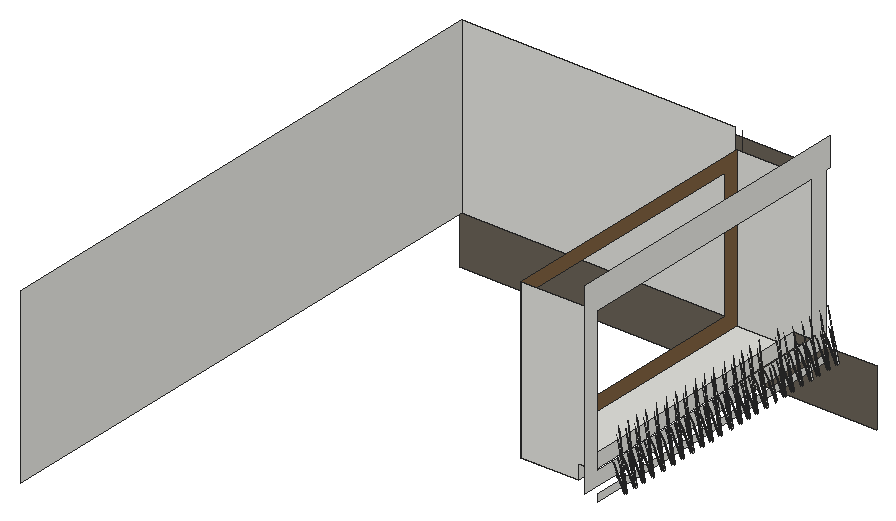
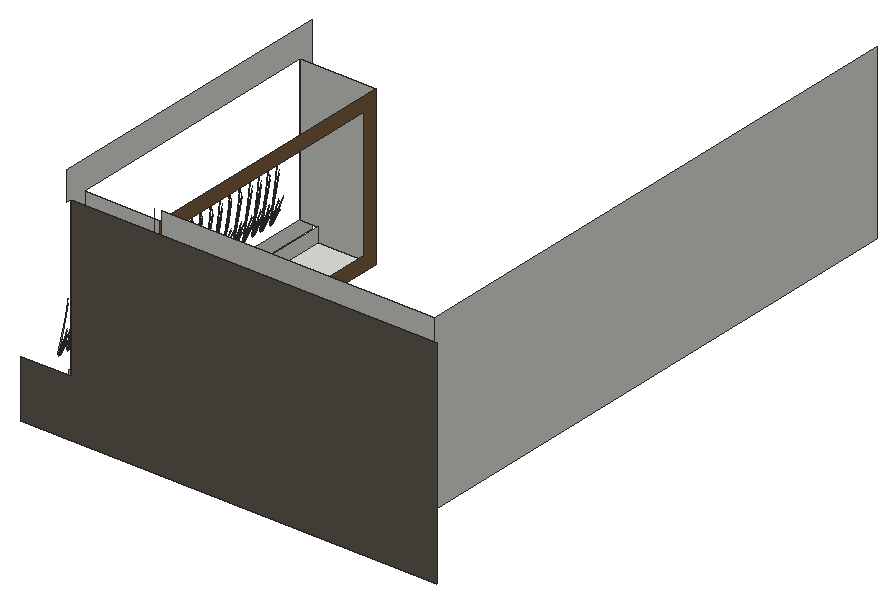
# SketchUp Ruby script. Lengths in inches.
U = 1.inch
M = Sketchup.active_model
def pt(a) = Geom::Point3d.new(a.map { |v| v * U })
def face(e, loops, mat)
  f = e.add_face(loops[0].map { |a| pt(a) })
  loops[1..].each { |l| e.add_face(l.map { |a| pt(a) }).erase! }
  f.material = f.back_material = mat if mat
  f
end
# faces: each face lists its corners as indices into pts; further lists are holes
def faces(e, pts, list, mat = nil) = list.each { |f| face(e, (f[0].is_a?(Array) ? f : [f]).map { |l| l.map { |i| pts[i] } }, mat) }
# xy, xz, yz: faces in a plane at the given z, y or x. An outline is a flat list of corners, or four numbers for a rectangle; further outlines are holes
def ring(l) = l.size == 4 ? [[l[0], l[1]], [l[2], l[1]], [l[2], l[3]], [l[0], l[3]]] : l.each_slice(2).to_a
def flat(e, list, mat, &to3) = list.each { |f| face(e, (f[0].is_a?(Array) ? f : [f]).map { |l| ring(l).map { |u, v| to3.(u, v) } }, mat) }
def xy(e, z, list, mat = nil) = flat(e, list, mat) { |x, y| [x, y, z] }
def xz(e, y, list, mat = nil) = flat(e, list, mat) { |x, z| [x, y, z] }
def yz(e, x, list, mat = nil) = flat(e, list, mat) { |y, z| [x, y, z] }
def lines(e, pts, list) = list.each { |a, b| e.add_line(pt(pts[a]), pt(pts[b])) }
# prism: a flat outline (further loops are holes) pulled along v
def prism(e, loops, v, mat = nil)
  f = face(e, loops, mat); d = Geom::Vector3d.new(v.map { |x| x * U })
  f.pushpull(f.normal.samedirection?(d) ? d.length : -d.length)
end
def box(e, o, s, mat = nil) = prism(e, [[o, [o[0] + s[0], o[1], o[2]], [o[0] + s[0], o[1] + s[1], o[2]], [o[0], o[1] + s[1], o[2]]]], [0, 0, s[2]], mat)
def at(x, y, z, deg = 0) = Geom::Transformation.translation(pt([x, y, z])) * Geom::Transformation.rotation(ORIGIN, Z_AXIS, deg.degrees)
def axes(o, x, y, z) = Geom::Transformation.new([*x, 0, *y, 0, *z, 0, *pt(o).to_a, 1])
def part(name) = M.definitions.add(name)
# library, detail: a bought-in or finely detailed component or shape, given as its bounding box
def library(name, o, s) = part(name).tap { |d| box(d.entities, o, s) }
def detail(e, o, s) = box(e.add_group.entities, o, s)
def put(e, d, t, mat = nil) = e.add_instance(d, t).tap { |i| i.material = mat if mat }
def group(e, t, mat = nil) = e.add_group.tap { |g| g.transformation = t; g.material = mat if mat }.entities
root = M.entities
M.materials.add("LightPink_Translucent").color = [144, 107, 117]
M.materials["LightPink_Translucent"].alpha = 0.75
M.materials.add("Plaster_04_1K").color = [106, 98, 87]
M.materials.add("Plywood_01_1K").color = [125, 96, 64]
c1 = part("blade")
p = [[2.15,0.21,22],[0,0.17,0],[0.09,0.45,0],[2.18,0.31,22],[2.29,0.31,22],[0.38,0.45,0],
  [2.48,0.24,33],[2.49,0.24,33],[2.48,0.22,33]]
faces(c1.entities,p,[[0,1,2,3],[4,5,2,3],[6,3,4,7],[8,0,3,6]])
c2 = part("seeds")
p = [[0.3,-0.1,1.38],[-0.01,-0.03,1.59],[-0.01,-0.03,0.03],[0.14,-0.07,-0.07],[0.29,-0.03,3],[0.15,0.01,3.11]]
faces(c2.entities,p,[[0,1,2,3],[1,0,4,5]],"LightPink_Translucent")
c3 = part("blade with seeds")
put(c3.entities,c1,at(0,0,0))
put(c3.entities,c2,axes([2.4,0.25,30.99],[1.5799,-0.05474,1.17369],[-0.12525,1.92788,0.29478],[-0.07173,-0.02425,1.56792]))
xy(root,48,[[247,274,295,499],[247,499,295,505]])
xz(root,274,[[247,48,247,180,310,180,310,60,295,60,295,48]])
xz(root,499,[[247,48,295,48,295,60,310,60,310,180,247,180]])
xz(root,505,[[13,48,241,192]])
xz(root,514,[[4,0,4,180,310,180,310,48,352,48,352,0]],"Plaster_04_1K")
yz(root,13,[[43,48,505,192]])
yz(root,247,[[[274,48,499,180],[286,60,487,168]]],"Plywood_01_1K")
yz(root,295,[[274,48,499,60]])
yz(root,310,[[262,48,514,48,514,180,499,180,499,60,274,60,274,180,518,180,518,204,262,204]])
yz(root,316,[[268,42,508,48]])
p = [[247,505,48],[241,505,48],[295,505,48],[304,505,48],[247,505,192]]
lines(root,p,[[0,1],[2,3],[4,0]])
put(root,c3,axes([331.07,277.47,50.29],[0.17547,0.03208,1.26356],[0.1131,0.32764,-0.27174],[-0.23835,0.06133,0.54024]))
put(root,c3,axes([331.07,287.27,50.29],[0.17547,0.03208,1.26356],[0.1131,0.32764,-0.27174],[-0.23835,0.06133,0.54024]))
put(root,c3,axes([331.07,296.25,50.29],[0.17547,0.03208,1.26356],[0.1131,0.32764,-0.27174],[-0.23835,0.06133,0.54024]))
put(root,c3,axes([331.07,305.73,50.29],[0.17547,0.03208,1.26356],[0.1131,0.32764,-0.27174],[-0.23835,0.06133,0.54024]))
put(root,c3,axes([331.07,316.72,50.29],[0.17547,0.03208,1.26356],[0.1131,0.32764,-0.27174],[-0.23835,0.06133,0.54024]))
put(root,c3,axes([331.07,327.32,50.29],[0.17547,0.03208,1.26356],[0.1131,0.32764,-0.27174],[-0.23835,0.06133,0.54024]))
put(root,c3,axes([331.07,337.02,50.29],[0.17547,0.03208,1.26356],[0.1131,0.32764,-0.27174],[-0.23835,0.06133,0.54024]))
put(root,c3,axes([331.07,346.96,50.29],[0.17547,0.03208,1.26356],[0.1131,0.32764,-0.27174],[-0.23835,0.06133,0.54024]))
put(root,c3,axes([331.07,357.68,50.29],[0.17547,0.03208,1.26356],[0.1131,0.32764,-0.27174],[-0.23835,0.06133,0.54024]))
put(root,c3,axes([331.07,367.01,50.29],[0.17547,0.03208,1.26356],[0.1131,0.32764,-0.27174],[-0.23835,0.06133,0.54024]))
put(root,c3,axes([331.07,376.48,50.29],[0.17547,0.03208,1.26356],[0.1131,0.32764,-0.27174],[-0.23835,0.06133,0.54024]))
put(root,c3,axes([331.07,387.79,50.29],[0.17547,0.03208,1.26356],[0.1131,0.32764,-0.27174],[-0.23835,0.06133,0.54024]))
put(root,c3,axes([331.07,397.47,50.29],[0.17547,0.03208,1.26356],[0.1131,0.32764,-0.27174],[-0.23835,0.06133,0.54024]))
put(root,c3,axes([331.07,405.93,50.29],[0.17547,0.03208,1.26356],[0.1131,0.32764,-0.27174],[-0.23835,0.06133,0.54024]))
put(root,c3,axes([331.07,414.4,50.29],[0.17547,0.03208,1.26356],[0.1131,0.32764,-0.27174],[-0.23835,0.06133,0.54024]))
put(root,c3,axes([331.07,424.29,50.29],[0.17547,0.03208,1.26356],[0.1131,0.32764,-0.27174],[-0.23835,0.06133,0.54024]))
put(root,c3,axes([331.07,443.68,50.29],[0.17547,0.03208,1.26356],[0.1131,0.32764,-0.27174],[-0.23835,0.06133,0.54024]))
put(root,c3,axes([331.07,452.05,50.29],[0.17547,0.03208,1.26356],[0.1131,0.32764,-0.27174],[-0.23835,0.06133,0.54024]))
put(root,c3,axes([331.07,461.57,50.29],[0.17547,0.03208,1.26356],[0.1131,0.32764,-0.27174],[-0.23835,0.06133,0.54024]))
put(root,c3,axes([331.07,471.125,50.29],[0.17547,0.03208,1.26356],[0.1131,0.32764,-0.27174],[-0.23835,0.06133,0.54024]))
put(root,c3,axes([331.07,478.92,50.29],[0.17547,0.03208,1.26356],[0.1131,0.32764,-0.27174],[-0.23835,0.06133,0.54024]))
put(root,c3,axes([331.07,489.62,50.29],[0.17547,0.03208,1.26356],[0.1131,0.32764,-0.27174],[-0.23835,0.06133,0.54024]))
put(root,c3,axes([331.07,498.4,50.29],[0.17547,0.03208,1.26356],[0.1131,0.32764,-0.27174],[-0.23835,0.06133,0.54024]))
put(root,c3,axes([331.74,275.88,50.29],[0.09858,0.10879,1.26356],[-0.22716,0.29571,-0.27174],[-0.23325,-0.07068,0.54024]))
put(root,c3,axes([331.74,285.6875,50.29],[0.09858,0.10879,1.26356],[-0.22716,0.29571,-0.27174],[-0.23325,-0.07068,0.54024]))
put(root,c3,axes([331.74,294.66,50.29],[0.09858,0.10879,1.26356],[-0.22716,0.29571,-0.27174],[-0.23325,-0.07068,0.54024]))
put(root,c3,axes([331.74,304.15,50.29],[0.09858,0.10879,1.26356],[-0.22716,0.29571,-0.27174],[-0.23325,-0.07068,0.54024]))
put(root,c3,axes([331.74,315.14,50.29],[0.09858,0.10879,1.26356],[-0.22716,0.29571,-0.27174],[-0.23325,-0.07068,0.54024]))
put(root,c3,axes([331.74,325.73,50.29],[0.09858,0.10879,1.26356],[-0.22716,0.29571,-0.27174],[-0.23325,-0.07068,0.54024]))
put(root,c3,axes([331.74,335.4375,50.29],[0.09858,0.10879,1.26356],[-0.22716,0.29571,-0.27174],[-0.23325,-0.07068,0.54024]))
put(root,c3,axes([331.74,345.375,50.29],[0.09858,0.10879,1.26356],[-0.22716,0.29571,-0.27174],[-0.23325,-0.07068,0.54024]))
put(root,c3,axes([331.74,356.1,50.29],[0.09858,0.10879,1.26356],[-0.22716,0.29571,-0.27174],[-0.23325,-0.07068,0.54024]))
put(root,c3,axes([331.74,365.42,50.29],[0.09858,0.10879,1.26356],[-0.22716,0.29571,-0.27174],[-0.23325,-0.07068,0.54024]))
put(root,c3,axes([331.74,374.89,50.29],[0.09858,0.10879,1.26356],[-0.22716,0.29571,-0.27174],[-0.23325,-0.07068,0.54024]))
put(root,c3,axes([331.74,386.2,50.29],[0.09858,0.10879,1.26356],[-0.22716,0.29571,-0.27174],[-0.23325,-0.07068,0.54024]))
put(root,c3,axes([331.74,395.88,50.29],[0.09858,0.10879,1.26356],[-0.22716,0.29571,-0.27174],[-0.23325,-0.07068,0.54024]))
put(root,c3,axes([331.74,404.35,50.29],[0.09858,0.10879,1.26356],[-0.22716,0.29571,-0.27174],[-0.23325,-0.07068,0.54024]))
put(root,c3,axes([331.74,412.8125,50.29],[0.09858,0.10879,1.26356],[-0.22716,0.29571,-0.27174],[-0.23325,-0.07068,0.54024]))
put(root,c3,axes([331.74,422.71,50.29],[0.09858,0.10879,1.26356],[-0.22716,0.29571,-0.27174],[-0.23325,-0.07068,0.54024]))
put(root,c3,axes([331.74,442.09,50.29],[0.09858,0.10879,1.26356],[-0.22716,0.29571,-0.27174],[-0.23325,-0.07068,0.54024]))
put(root,c3,axes([331.74,450.47,50.29],[0.09858,0.10879,1.26356],[-0.22716,0.29571,-0.27174],[-0.23325,-0.07068,0.54024]))
put(root,c3,axes([331.74,459.98,50.29],[0.09858,0.10879,1.26356],[-0.22716,0.29571,-0.27174],[-0.23325,-0.07068,0.54024]))
put(root,c3,axes([331.74,469.54,50.29],[0.09858,0.10879,1.26356],[-0.22716,0.29571,-0.27174],[-0.23325,-0.07068,0.54024]))
put(root,c3,axes([331.74,477.33,50.29],[0.09858,0.10879,1.26356],[-0.22716,0.29571,-0.27174],[-0.23325,-0.07068,0.54024]))
put(root,c3,axes([331.74,488.03,50.29],[0.09858,0.10879,1.26356],[-0.22716,0.29571,-0.27174],[-0.23325,-0.07068,0.54024]))
put(root,c3,axes([331.74,496.8125,50.29],[0.09858,0.10879,1.26356],[-0.22716,0.29571,-0.27174],[-0.23325,-0.07068,0.54024]))
put(root,c3,axes([331.39,276.61,49.32],[0.0128,0.06158,1.55816],[-0.25814,0.3216,-0.23804],[-0.18336,-0.01621,0.26541]))
put(root,c3,axes([331.39,286.42,49.32],[0.0128,0.06158,1.55816],[-0.25814,0.3216,-0.23804],[-0.18336,-0.01621,0.26541]))
put(root,c3,axes([331.39,295.39,49.32],[0.0128,0.06158,1.55816],[-0.25814,0.3216,-0.23804],[-0.18336,-0.01621,0.26541]))
put(root,c3,axes([331.39,304.875,49.32],[0.0128,0.06158,1.55816],[-0.25814,0.3216,-0.23804],[-0.18336,-0.01621,0.26541]))
put(root,c3,axes([331.39,315.87,49.32],[0.0128,0.06158,1.55816],[-0.25814,0.3216,-0.23804],[-0.18336,-0.01621,0.26541]))
put(root,c3,axes([331.39,326.46,49.32],[0.0128,0.06158,1.55816],[-0.25814,0.3216,-0.23804],[-0.18336,-0.01621,0.26541]))
put(root,c3,axes([331.39,336.17,49.32],[0.0128,0.06158,1.55816],[-0.25814,0.3216,-0.23804],[-0.18336,-0.01621,0.26541]))
put(root,c3,axes([331.39,346.1,49.32],[0.0128,0.06158,1.55816],[-0.25814,0.3216,-0.23804],[-0.18336,-0.01621,0.26541]))
put(root,c3,axes([331.39,356.83,49.32],[0.0128,0.06158,1.55816],[-0.25814,0.3216,-0.23804],[-0.18336,-0.01621,0.26541]))
put(root,c3,axes([331.39,366.15,49.32],[0.0128,0.06158,1.55816],[-0.25814,0.3216,-0.23804],[-0.18336,-0.01621,0.26541]))
put(root,c3,axes([331.39,375.625,49.32],[0.0128,0.06158,1.55816],[-0.25814,0.3216,-0.23804],[-0.18336,-0.01621,0.26541]))
put(root,c3,axes([331.39,386.93,49.32],[0.0128,0.06158,1.55816],[-0.25814,0.3216,-0.23804],[-0.18336,-0.01621,0.26541]))
put(root,c3,axes([331.39,396.61,49.32],[0.0128,0.06158,1.55816],[-0.25814,0.3216,-0.23804],[-0.18336,-0.01621,0.26541]))
put(root,c3,axes([331.39,405.07,49.32],[0.0128,0.06158,1.55816],[-0.25814,0.3216,-0.23804],[-0.18336,-0.01621,0.26541]))
put(root,c3,axes([331.39,413.54,49.32],[0.0128,0.06158,1.55816],[-0.25814,0.3216,-0.23804],[-0.18336,-0.01621,0.26541]))
put(root,c3,axes([331.39,423.4375,49.32],[0.0128,0.06158,1.55816],[-0.25814,0.3216,-0.23804],[-0.18336,-0.01621,0.26541]))
put(root,c3,axes([331.39,442.82,49.32],[0.0128,0.06158,1.55816],[-0.25814,0.3216,-0.23804],[-0.18336,-0.01621,0.26541]))
put(root,c3,axes([331.39,451.2,49.32],[0.0128,0.06158,1.55816],[-0.25814,0.3216,-0.23804],[-0.18336,-0.01621,0.26541]))
put(root,c3,axes([331.39,460.71,49.32],[0.0128,0.06158,1.55816],[-0.25814,0.3216,-0.23804],[-0.18336,-0.01621,0.26541]))
put(root,c3,axes([331.39,470.27,49.32],[0.0128,0.06158,1.55816],[-0.25814,0.3216,-0.23804],[-0.18336,-0.01621,0.26541]))
put(root,c3,axes([331.39,478.0625,49.32],[0.0128,0.06158,1.55816],[-0.25814,0.3216,-0.23804],[-0.18336,-0.01621,0.26541]))
put(root,c3,axes([331.39,488.76,49.32],[0.0128,0.06158,1.55816],[-0.25814,0.3216,-0.23804],[-0.18336,-0.01621,0.26541]))
put(root,c3,axes([331.39,497.54,49.32],[0.0128,0.06158,1.55816],[-0.25814,0.3216,-0.23804],[-0.18336,-0.01621,0.26541]))
put(root,c3,axes([330.7,278.16,50.44],[0.21042,-0.1771,1.01491],[0.08303,0.28036,0.74569],[-0.15207,0.0502,0.22354]))
put(root,c3,axes([332.65,433.8125,50.29],[0.17547,0.03208,1.26356],[0.1131,0.32764,-0.27174],[-0.23835,0.06133,0.54024]))
put(root,c3,axes([331.25,278.34,49.32],[0.06773,0.03904,1.55816],[0.11484,0.36171,-0.23804],[-0.15011,0.07713,0.26541]))
put(root,c3,axes([331.25,288.14,49.32],[0.06773,0.03904,1.55816],[0.11484,0.36171,-0.23804],[-0.15011,0.07713,0.26541]))
put(root,c3,axes([331.25,297.12,49.32],[0.06773,0.03904,1.55816],[0.11484,0.36171,-0.23804],[-0.15011,0.07713,0.26541]))
put(root,c3,axes([331.25,306.6,49.32],[0.06773,0.03904,1.55816],[0.11484,0.36171,-0.23804],[-0.15011,0.07713,0.26541]))
put(root,c3,axes([331.25,317.59,49.32],[0.06773,0.03904,1.55816],[0.11484,0.36171,-0.23804],[-0.15011,0.07713,0.26541]))
put(root,c3,axes([331.25,328.1875,49.32],[0.06773,0.03904,1.55816],[0.11484,0.36171,-0.23804],[-0.15011,0.07713,0.26541]))
put(root,c3,axes([331.25,337.89,49.32],[0.06773,0.03904,1.55816],[0.11484,0.36171,-0.23804],[-0.15011,0.07713,0.26541]))
put(root,c3,axes([331.25,347.83,49.32],[0.06773,0.03904,1.55816],[0.11484,0.36171,-0.23804],[-0.15011,0.07713,0.26541]))
put(root,c3,axes([331.25,358.55,49.32],[0.06773,0.03904,1.55816],[0.11484,0.36171,-0.23804],[-0.15011,0.07713,0.26541]))
put(root,c3,axes([331.25,367.875,49.32],[0.06773,0.03904,1.55816],[0.11484,0.36171,-0.23804],[-0.15011,0.07713,0.26541]))
put(root,c3,axes([331.25,377.35,49.32],[0.06773,0.03904,1.55816],[0.11484,0.36171,-0.23804],[-0.15011,0.07713,0.26541]))
put(root,c3,axes([331.25,388.66,49.32],[0.06773,0.03904,1.55816],[0.11484,0.36171,-0.23804],[-0.15011,0.07713,0.26541]))
put(root,c3,axes([331.25,398.34,49.32],[0.06773,0.03904,1.55816],[0.11484,0.36171,-0.23804],[-0.15011,0.07713,0.26541]))
put(root,c3,axes([331.25,406.8,49.32],[0.06773,0.03904,1.55816],[0.11484,0.36171,-0.23804],[-0.15011,0.07713,0.26541]))
put(root,c3,axes([331.25,415.27,49.32],[0.06773,0.03904,1.55816],[0.11484,0.36171,-0.23804],[-0.15011,0.07713,0.26541]))
put(root,c3,axes([331.25,425.16,49.32],[0.06773,0.03904,1.55816],[0.11484,0.36171,-0.23804],[-0.15011,0.07713,0.26541]))
put(root,c3,axes([331.25,444.55,49.32],[0.06773,0.03904,1.55816],[0.11484,0.36171,-0.23804],[-0.15011,0.07713,0.26541]))
put(root,c3,axes([331.25,452.92,49.32],[0.06773,0.03904,1.55816],[0.11484,0.36171,-0.23804],[-0.15011,0.07713,0.26541]))
put(root,c3,axes([331.25,462.4375,49.32],[0.06773,0.03904,1.55816],[0.11484,0.36171,-0.23804],[-0.15011,0.07713,0.26541]))
put(root,c3,axes([331.25,471.99,49.32],[0.06773,0.03904,1.55816],[0.11484,0.36171,-0.23804],[-0.15011,0.07713,0.26541]))
put(root,c3,axes([331.25,479.79,49.32],[0.06773,0.03904,1.55816],[0.11484,0.36171,-0.23804],[-0.15011,0.07713,0.26541]))
put(root,c3,axes([331.25,490.49,49.32],[0.06773,0.03904,1.55816],[0.11484,0.36171,-0.23804],[-0.15011,0.07713,0.26541]))
put(root,c3,axes([331.25,499.27,49.32],[0.06773,0.03904,1.55816],[0.11484,0.36171,-0.23804],[-0.15011,0.07713,0.26541]))
put(root,c3,axes([331.16,276.21,50.44],[0.32236,-0.02796,1.01491],[-0.20448,0.24636,0.74569],[-0.1593,-0.03696,0.22354]))
put(root,c3,axes([333.33,432.23,50.29],[0.09858,0.10879,1.26356],[-0.22716,0.29571,-0.27174],[-0.23325,-0.07068,0.54024]))
put(root,c3,axes([333.08,277.17,49.82],[-0.52523,-0.06406,-0.55095],[0.11084,-0.39517,-0.1446],[-0.15674,-0.04788,1.21613]))
put(root,c3,axes([333.08,286.97,49.82],[-0.52523,-0.06406,-0.55095],[0.11084,-0.39517,-0.1446],[-0.15674,-0.04788,1.21613]))
put(root,c3,axes([333.08,295.95,49.82],[-0.52523,-0.06406,-0.55095],[0.11084,-0.39517,-0.1446],[-0.15674,-0.04788,1.21613]))
put(root,c3,axes([333.08,305.43,49.82],[-0.52523,-0.06406,-0.55095],[0.11084,-0.39517,-0.1446],[-0.15674,-0.04788,1.21613]))
put(root,c3,axes([333.08,316.42,49.82],[-0.52523,-0.06406,-0.55095],[0.11084,-0.39517,-0.1446],[-0.15674,-0.04788,1.21613]))
put(root,c3,axes([333.08,327.02,49.82],[-0.52523,-0.06406,-0.55095],[0.11084,-0.39517,-0.1446],[-0.15674,-0.04788,1.21613]))
put(root,c3,axes([333.08,336.73,49.82],[-0.52523,-0.06406,-0.55095],[0.11084,-0.39517,-0.1446],[-0.15674,-0.04788,1.21613]))
put(root,c3,axes([333.08,346.66,49.82],[-0.52523,-0.06406,-0.55095],[0.11084,-0.39517,-0.1446],[-0.15674,-0.04788,1.21613]))
put(root,c3,axes([333.08,357.38,49.82],[-0.52523,-0.06406,-0.55095],[0.11084,-0.39517,-0.1446],[-0.15674,-0.04788,1.21613]))
put(root,c3,axes([333.08,366.71,49.82],[-0.52523,-0.06406,-0.55095],[0.11084,-0.39517,-0.1446],[-0.15674,-0.04788,1.21613]))
put(root,c3,axes([333.08,376.18,49.82],[-0.52523,-0.06406,-0.55095],[0.11084,-0.39517,-0.1446],[-0.15674,-0.04788,1.21613]))
put(root,c3,axes([333.08,387.49,49.82],[-0.52523,-0.06406,-0.55095],[0.11084,-0.39517,-0.1446],[-0.15674,-0.04788,1.21613]))
put(root,c3,axes([333.08,397.17,49.82],[-0.52523,-0.06406,-0.55095],[0.11084,-0.39517,-0.1446],[-0.15674,-0.04788,1.21613]))
put(root,c3,axes([333.08,405.63,49.82],[-0.52523,-0.06406,-0.55095],[0.11084,-0.39517,-0.1446],[-0.15674,-0.04788,1.21613]))
put(root,c3,axes([333.08,414.1,49.82],[-0.52523,-0.06406,-0.55095],[0.11084,-0.39517,-0.1446],[-0.15674,-0.04788,1.21613]))
put(root,c3,axes([333.08,424,49.82],[-0.52523,-0.06406,-0.55095],[0.11084,-0.39517,-0.1446],[-0.15674,-0.04788,1.21613]))
put(root,c3,axes([333.08,443.38,49.82],[-0.52523,-0.06406,-0.55095],[0.11084,-0.39517,-0.1446],[-0.15674,-0.04788,1.21613]))
put(root,c3,axes([333.08,451.75,49.82],[-0.52523,-0.06406,-0.55095],[0.11084,-0.39517,-0.1446],[-0.15674,-0.04788,1.21613]))
put(root,c3,axes([333.08,461.27,49.82],[-0.52523,-0.06406,-0.55095],[0.11084,-0.39517,-0.1446],[-0.15674,-0.04788,1.21613]))
put(root,c3,axes([333.08,470.83,49.82],[-0.52523,-0.06406,-0.55095],[0.11084,-0.39517,-0.1446],[-0.15674,-0.04788,1.21613]))
put(root,c3,axes([333.08,478.62,49.82],[-0.52523,-0.06406,-0.55095],[0.11084,-0.39517,-0.1446],[-0.15674,-0.04788,1.21613]))
put(root,c3,axes([333.08,489.32,49.82],[-0.52523,-0.06406,-0.55095],[0.11084,-0.39517,-0.1446],[-0.15674,-0.04788,1.21613]))
put(root,c3,axes([333.08,498.1,49.82],[-0.52523,-0.06406,-0.55095],[0.11084,-0.39517,-0.1446],[-0.15674,-0.04788,1.21613]))
put(root,c3,axes([332.98,432.96,49.32],[0.0128,0.06158,1.55816],[-0.25814,0.3216,-0.23804],[-0.18336,-0.01621,0.26541]))
put(root,c3,axes([332.39,277.92,49.78],[-0.47255,-0.19538,-0.43871],[0.28245,-0.35034,0],[-0.10763,-0.0445,1.3917]))
put(root,c3,axes([332.39,287.72,49.78],[-0.47255,-0.19538,-0.43871],[0.28245,-0.35034,0],[-0.10763,-0.0445,1.3917]))
put(root,c3,axes([332.39,296.7,49.78],[-0.47255,-0.19538,-0.43871],[0.28245,-0.35034,0],[-0.10763,-0.0445,1.3917]))
put(root,c3,axes([332.39,306.18,49.78],[-0.47255,-0.19538,-0.43871],[0.28245,-0.35034,0],[-0.10763,-0.0445,1.3917]))
put(root,c3,axes([332.39,317.17,49.78],[-0.47255,-0.19538,-0.43871],[0.28245,-0.35034,0],[-0.10763,-0.0445,1.3917]))
put(root,c3,axes([332.39,327.77,49.78],[-0.47255,-0.19538,-0.43871],[0.28245,-0.35034,0],[-0.10763,-0.0445,1.3917]))
put(root,c3,axes([332.39,337.47,49.78],[-0.47255,-0.19538,-0.43871],[0.28245,-0.35034,0],[-0.10763,-0.0445,1.3917]))
put(root,c3,axes([332.39,347.41,49.78],[-0.47255,-0.19538,-0.43871],[0.28245,-0.35034,0],[-0.10763,-0.0445,1.3917]))
put(root,c3,axes([332.39,358.13,49.78],[-0.47255,-0.19538,-0.43871],[0.28245,-0.35034,0],[-0.10763,-0.0445,1.3917]))
put(root,c3,axes([332.39,367.46,49.78],[-0.47255,-0.19538,-0.43871],[0.28245,-0.35034,0],[-0.10763,-0.0445,1.3917]))
put(root,c3,axes([332.39,376.93,49.78],[-0.47255,-0.19538,-0.43871],[0.28245,-0.35034,0],[-0.10763,-0.0445,1.3917]))
put(root,c3,axes([332.39,388.24,49.78],[-0.47255,-0.19538,-0.43871],[0.28245,-0.35034,0],[-0.10763,-0.0445,1.3917]))
put(root,c3,axes([332.39,397.92,49.78],[-0.47255,-0.19538,-0.43871],[0.28245,-0.35034,0],[-0.10763,-0.0445,1.3917]))
put(root,c3,axes([332.39,406.38,49.78],[-0.47255,-0.19538,-0.43871],[0.28245,-0.35034,0],[-0.10763,-0.0445,1.3917]))
put(root,c3,axes([332.39,414.85,49.78],[-0.47255,-0.19538,-0.43871],[0.28245,-0.35034,0],[-0.10763,-0.0445,1.3917]))
put(root,c3,axes([332.39,424.74,49.78],[-0.47255,-0.19538,-0.43871],[0.28245,-0.35034,0],[-0.10763,-0.0445,1.3917]))
put(root,c3,axes([332.39,444.13,49.78],[-0.47255,-0.19538,-0.43871],[0.28245,-0.35034,0],[-0.10763,-0.0445,1.3917]))
